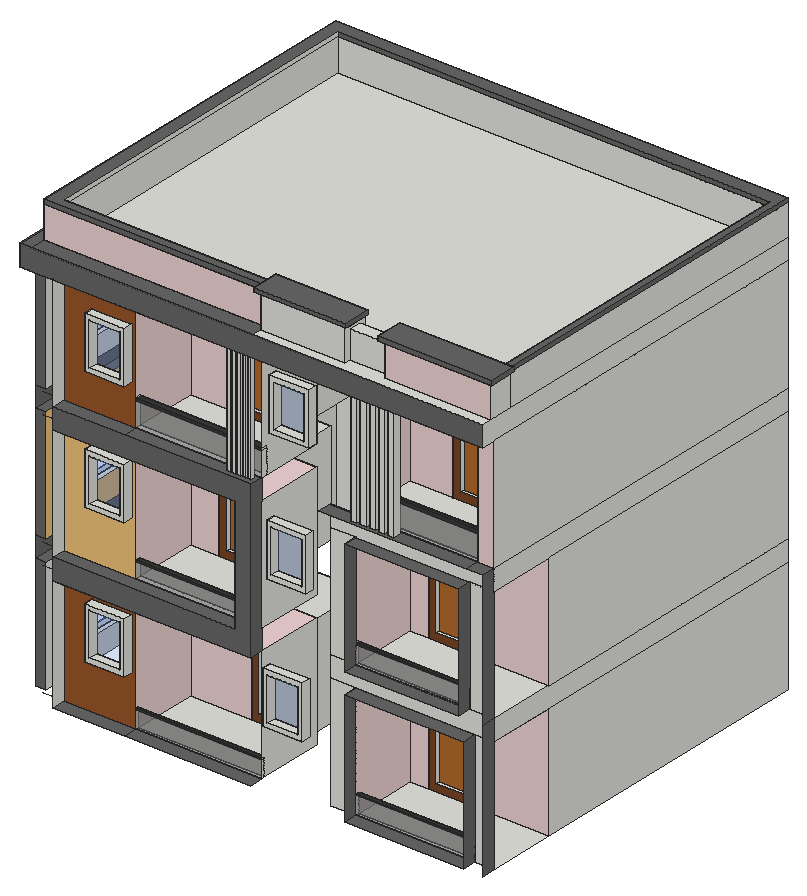
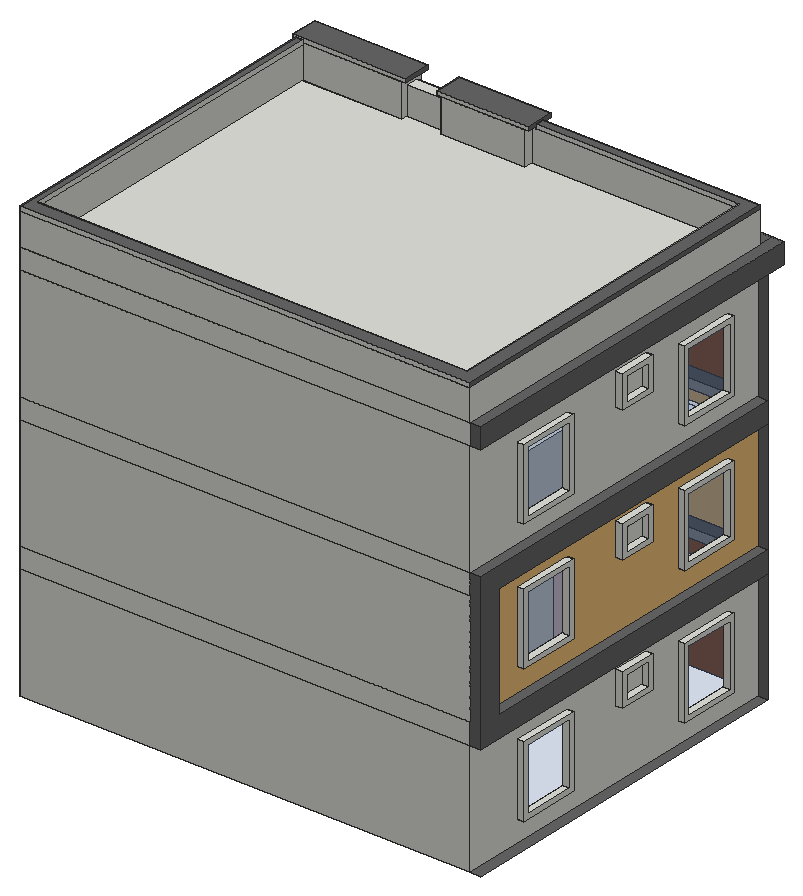
# SketchUp Ruby script. Lengths in inches.
U = 1.inch
M = Sketchup.active_model
def pt(a) = Geom::Point3d.new(a.map { |v| v * U })
def face(e, loops, mat)
  f = e.add_face(loops[0].map { |a| pt(a) })
  loops[1..].each { |l| e.add_face(l.map { |a| pt(a) }).erase! }
  f.material = f.back_material = mat if mat
  f
end
# faces: each face lists its corners as indices into pts; further lists are holes
def faces(e, pts, list, mat = nil) = list.each { |f| face(e, (f[0].is_a?(Array) ? f : [f]).map { |l| l.map { |i| pts[i] } }, mat) }
# xy, xz, yz: faces in a plane at the given z, y or x. An outline is a flat list of corners, or four numbers for a rectangle; further outlines are holes
def ring(l) = l.size == 4 ? [[l[0], l[1]], [l[2], l[1]], [l[2], l[3]], [l[0], l[3]]] : l.each_slice(2).to_a
def flat(e, list, mat, &to3) = list.each { |f| face(e, (f[0].is_a?(Array) ? f : [f]).map { |l| ring(l).map { |u, v| to3.(u, v) } }, mat) }
def xy(e, z, list, mat = nil) = flat(e, list, mat) { |x, y| [x, y, z] }
def xz(e, y, list, mat = nil) = flat(e, list, mat) { |x, z| [x, y, z] }
def yz(e, x, list, mat = nil) = flat(e, list, mat) { |y, z| [x, y, z] }
def lines(e, pts, list) = list.each { |a, b| e.add_line(pt(pts[a]), pt(pts[b])) }
# prism: a flat outline (further loops are holes) pulled along v
def prism(e, loops, v, mat = nil)
  f = face(e, loops, mat); d = Geom::Vector3d.new(v.map { |x| x * U })
  f.pushpull(f.normal.samedirection?(d) ? d.length : -d.length)
end
def box(e, o, s, mat = nil) = prism(e, [[o, [o[0] + s[0], o[1], o[2]], [o[0] + s[0], o[1] + s[1], o[2]], [o[0], o[1] + s[1], o[2]]]], [0, 0, s[2]], mat)
def at(x, y, z, deg = 0) = Geom::Transformation.translation(pt([x, y, z])) * Geom::Transformation.rotation(ORIGIN, Z_AXIS, deg.degrees)
def axes(o, x, y, z) = Geom::Transformation.new([*x, 0, *y, 0, *z, 0, *pt(o).to_a, 1])
def part(name) = M.definitions.add(name)
# library, detail: a bought-in or finely detailed component or shape, given as its bounding box
def library(name, o, s) = part(name).tap { |d| box(d.entities, o, s) }
def detail(e, o, s) = box(e.add_group.entities, o, s)
def put(e, d, t, mat = nil) = e.add_instance(d, t).tap { |i| i.material = mat if mat }
def group(e, t, mat = nil) = e.add_group.tap { |g| g.transformation = t; g.material = mat if mat }.entities
root = M.entities
M.materials.add("Generic").color = [103, 103, 103]
M.materials.add("Generic\#1").color = [239, 210, 210]
M.materials.add("[Color M07]").color = [58, 58, 58]
M.materials.add("[Translucent Glass Blue]").color = [98, 147, 234]
M.materials["[Translucent Glass Blue]"].alpha = 0.25
M.materials.add("[Translucent Glass Gray]").color = [128, 128, 128]
M.materials["[Translucent Glass Gray]"].alpha = 0.5
M.materials.add("[Wood Bamboo]").color = [177, 105, 43]
M.materials.add("[Wood Cherry Original]").color = [152, 86, 42]
M.materials.add("[Wood OSB]").color = [240, 195, 122]
M.materials.add("[Wood Veneer 01]").color = [120, 70, 37]
c1 = part("Group\#1")
xy(c1.entities,0,[[0,0,76.25,8.9375]])
xy(c1.entities,11.01,[[11.01,0,65.24,5.9375]])
xy(c1.entities,138.8,[[11.01,0,65.24,5.9375]])
xy(c1.entities,149.8125,[[0,0,76.25,8.9375]])
xz(c1.entities,0,[[[0,0,76.25,149.8125],[11.01,11.01,65.24,138.8]]],"[Wood Veneer 01]")
xz(c1.entities,5.9375,[[11.01,11.01,65.24,138.8]],"[Wood Bamboo]")
xz(c1.entities,8.9375,[[0,0,76.25,149.8125]])
yz(c1.entities,0,[[0,0,8.9375,149.8125]])
yz(c1.entities,11.01,[[0,11.01,5.9375,138.8]])
yz(c1.entities,65.24,[[0,11.01,5.9375,138.8]])
yz(c1.entities,76.25,[[0,0,8.9375,149.8125]])
xy(root,595.875,[[461.64,66.43,647.41,70.56],[785.17,66.43,960.48,72.06],[960.48,66.43,960.48,72.06,785.17,72.06,785.17,167.12,989.0625,167.12,989.0625,66.43],[461.64,70.56,461.64,167.12,551.875,167.12,551.875,277.93,628.125,277.93,628.125,167.12,647.41,167.12,647.41,70.56],[812,167.12,888.25,277.93]])
xy(root,595.875,[[356.25,45.93,461.64,66.43],[461.64,45.93,647.41,66.43],[785.17,45.93,960.48,66.43],[307.875,73.93,323.875,606.43]],"Generic")
xy(root,621.1875,[[461.64,66.43,647.41,70.56]])
xy(root,622.3125,[[785.17,66.43,960.48,72.06]])
xy(root,623.75,[[461.64,66.43,647.41,70.56]],"[Color M07]")
xy(root,624.6875,[[785.17,66.43,960.48,72.06]],"[Color M07]")
xy(root,627.86,[[313.8125,129.65,323.875,221.17],[313.8125,426.9,323.875,518.42]])
xy(root,634.68,[[313.8125,136.47,323.875,214.35],[313.8125,433.72,323.875,511.6]])
xy(root,668.22,[[397.09,53.18,455.09,66.43]])
xy(root,674.73,[[403.59,53.18,448.59,66.43]])
xy(root,675.14,[[659.17,53.18,717.17,66.43]])
xy(root,681.64,[[665.67,53.18,710.67,66.43]])
xy(root,698.74,[[312.6875,281.29,323.875,336.99]])
xy(root,705.5625,[[312.6875,288.11,323.875,330.17]])
xy(root,726.68,[[313.8125,136.47,323.875,214.35],[313.8125,433.72,323.875,511.6]])
xy(root,733.5,[[313.8125,129.65,323.875,221.17],[313.8125,426.9,323.875,518.42]])
xy(root,738.35,[[403.59,53.18,448.59,66.43]])
xy(root,740.25,[[312.6875,288.11,323.875,330.17]])
xy(root,744.6875,[[551.875,167.12,628.125,277.93],[812,167.12,888.25,277.93]])
xy(root,744.85,[[397.09,53.18,455.09,66.43]])
xy(root,745.27,[[665.67,53.18,710.67,66.43]])
xy(root,747.07,[[312.6875,281.29,323.875,336.99]])
xy(root,751.77,[[659.17,53.18,717.17,66.43]])
xy(root,763.875,[[356.25,45.93,647.41,66.43],[785.17,45.93,960.48,66.43],[307.875,73.93,323.875,606.43]],"Generic")
xy(root,763.875,[[461.64,66.43,647.41,167.12],[785.17,66.43,989.0625,167.12]],"Generic\#1")
xy(root,794.5,[[461.64,66.43,623.41,73.18],[623.41,66.43,623.41,73.18,461.64,73.18,461.64,167.12,503.75,167.12,503.75,277.93,580,277.93,580,167.12,647.41,167.12,647.41,66.43],[785.17,66.43,952.9375,71.18],[952.9375,66.43,952.9375,71.18,785.17,71.18,785.17,167.12,812,167.12,812,277.93,888.25,277.93,888.25,167.12,989.0625,167.12,989.0625,66.43]])
xy(root,794.5,[[356.25,45.93,623.41,66.43],[785.17,45.93,952.9375,66.43],[307.875,73.93,323.875,571.93]],"Generic")
xy(root,816,[[461.64,66.43,623.41,73.18]])
xy(root,819,[[461.64,66.43,623.41,73.18]],"[Color M07]")
xy(root,820.9375,[[785.17,66.43,952.9375,71.18]])
xy(root,823.3125,[[785.17,66.43,952.9375,71.18]],"[Color M07]")
xy(root,830.36,[[313.8125,129.65,323.875,221.17],[313.8125,426.9,323.875,518.42]])
xy(root,837.18,[[313.8125,136.47,323.875,214.35],[313.8125,433.72,323.875,511.6]])
xy(root,871.85,[[397.09,53.18,455.09,66.43],[664.84,53.18,722.84,66.43]])
xy(root,878.35,[[403.59,53.18,448.59,66.43],[671.34,53.18,716.34,66.43]])
xy(root,895.49,[[312.6875,281.29,323.875,336.99]])
xy(root,902.3125,[[312.6875,288.11,323.875,330.17]])
xy(root,929.18,[[313.8125,136.47,323.875,214.35],[313.8125,433.72,323.875,511.6]])
xy(root,936,[[313.8125,129.65,323.875,221.17],[313.8125,426.9,323.875,518.42]])
xy(root,937,[[312.6875,288.11,323.875,330.17]])
xy(root,941.98,[[403.59,53.18,448.59,66.43],[671.34,53.18,716.34,66.43]])
xy(root,943.82,[[312.6875,281.29,323.875,336.99]])
xy(root,944.3125,[[503.75,167.12,580,277.93],[812,167.12,888.25,277.93]])
xy(root,948.48,[[397.09,53.18,455.09,66.43],[664.84,53.18,722.84,66.43]])
xy(root,962.5,[[356.25,45.93,461.64,66.43],[461.64,45.93,623.41,66.43],[785.17,45.93,952.9375,66.43],[307.875,73.93,323.875,571.93]],"Generic")
xy(root,962.5,[[461.64,66.43,647.41,167.12],[785.17,66.43,989.0625,167.12]],"Generic\#1")
xy(root,993.125,[[461.64,66.43,647.41,74.74],[785.17,66.43,965.0625,71.74],[785.17,71.74,965.0625,167.12],[461.64,74.74,461.64,167.12,530.87,167.12,530.87,277.93,607.12,277.93,607.12,167.12,647.41,167.12,647.41,74.74],[848.37,167.12,924.62,277.93]])
xy(root,993.125,[[356.25,45.93,461.64,66.43],[[461.64,45.93,647.41,66.43],[635.77,54.52,641.21,59.96],[628.08,54.52,633.52,59.96],[620.39,54.52,625.83,59.96],[612.71,54.52,618.14,59.96],[605.02,54.52,610.46,59.96]],[[748.05,45.93,965.0625,66.43],[790.64,51.09,800.01,62.22],[804.2,51.09,813.58,62.22],[817.76,51.09,827.14,62.22],[831.33,51.09,840.7,62.22],[844.89,51.09,854.26,62.22]],[965.0625,45.93,989.0625,66.43],[307.875,73.93,323.875,606.43]],"Generic")
xy(root,1022.3,[[313.8125,129.65,323.875,221.17],[313.8125,426.9,323.875,518.42]])
xy(root,1028.5,[[461.64,66.43,647.41,74.74]])
xy(root,1029.12,[[313.8125,136.47,323.875,214.35],[313.8125,433.72,323.875,511.6]])
xy(root,1030.25,[[785.17,66.43,965.0625,71.74]])
xy(root,1032.5625,[[461.64,66.43,647.41,74.74]],"[Color M07]")
xy(root,1035.25,[[785.17,66.43,965.0625,71.74]],"[Color M07]")
xy(root,1050.97,[[397.09,53.18,455.09,66.43]])
xy(root,1057.48,[[403.59,53.18,448.59,66.43]])
xy(root,1064.99,[[668.28,53.18,726.28,66.43]])
xy(root,1071.5,[[674.78,53.18,719.78,66.43]])
xy(root,1094.49,[[312.6875,281.29,323.875,336.99]])
xy(root,1101.3125,[[312.6875,288.11,323.875,330.17]])
xy(root,1121.1,[[403.59,53.18,448.59,66.43]])
xy(root,1121.12,[[313.8125,136.47,323.875,214.35],[313.8125,433.72,323.875,511.6]])
xy(root,1127.6,[[397.09,53.18,455.09,66.43]])
xy(root,1127.9375,[[313.8125,129.65,323.875,221.17],[313.8125,426.9,323.875,518.42]])
xy(root,1135.12,[[674.78,53.18,719.78,66.43]])
xy(root,1136,[[312.6875,288.11,323.875,330.17]])
xy(root,1141.625,[[668.28,53.18,726.28,66.43]])
xy(root,1142.82,[[312.6875,281.29,323.875,336.99]])
xy(root,1142.9375,[[530.87,167.12,607.12,277.93],[848.37,167.12,924.62,277.93]])
xy(root,1161.125,[[307.875,45.93,323.875,73.93],[323.875,45.93,323.875,606.43,989.0625,606.43,989.0625,66.43,965.0625,66.43,965.0625,167.12,785.17,167.12,785.17,66.43,647.41,66.43,647.41,167.12,461.64,167.12,461.64,66.43,356.25,66.43,356.25,45.93],[790.64,45.93,800.01,51.09],[804.2,45.93,813.58,51.09],[817.76,45.93,827.14,51.09],
  [831.33,45.93,840.7,51.09],[844.89,45.93,854.26,51.09],[965.0625,45.93,989.0625,66.43],[790.64,51.09,800.01,62.22],[804.2,51.09,813.58,62.22],
  [817.76,51.09,827.14,62.22],[831.33,51.09,840.7,62.22],[844.89,51.09,854.26,62.22]])
xy(root,1161.125,[[356.25,45.93,461.64,66.43],[647.41,45.93,785.17,66.43],[307.875,73.93,323.875,606.43]],"Generic")
xy(root,1161.125,[[[461.64,45.93,647.41,167.12],[635.77,54.52,641.21,59.96],[628.08,54.52,633.52,59.96],[620.39,54.52,625.83,59.96],[612.71,54.52,618.14,59.96],[605.02,54.52,610.46,59.96]],[785.17,45.93,785.17,167.12,965.0625,167.12,965.0625,45.93,854.26,45.93,854.26,62.22,844.89,62.22,844.89,45.93,840.7,45.93,840.7,62.22,831.33,62.22,831.33,45.93,827.14,45.93,827.14,62.22,817.76,62.22,817.76,45.93,813.58,45.93,813.58,62.22,804.2,62.22,804.2,45.93,800.01,45.93,800.01,62.22,790.64,62.22,790.64,45.93]],"Generic\#1")
xy(root,1191.75,[[650.17,45.93,650.17,60.43,774.86,60.43,774.86,68.81,832.36,68.81,832.36,60.43,989.0625,60.43,989.0625,45.93],[650.17,60.43,774.86,95.68],[832.36,60.43,989.0625,95.68],[774.86,68.81,832.36,69.93],[323.875,69.93,323.875,606.43,989.0625,606.43,989.0625,95.68,979.4375,95.68,979.4375,586.43,343.5625,586.43,343.5625,82.81,650.17,82.81,650.17,69.93],
  [774.86,69.93,832.36,87.3],[343.5625,82.81,650.17,82.81,650.17,95.68,774.86,95.68,774.86,87.3,832.36,87.3,832.36,95.68,979.4375,95.68,979.4375,586.43,343.5625,586.43]])
xy(root,1191.75,[[307.875,45.93,323.875,606.43],[323.875,45.93,650.17,69.93]],"Generic")
xy(root,1233.18,[[774.86,68.81,832.36,87.3]])
xy(root,1238.5625,[[323.875,69.93,323.875,606.43,989.0625,606.43,989.0625,95.68,979.4375,95.68,979.4375,586.43,343.5625,586.43,343.5625,82.81,644.54,82.81,644.54,69.93]])
xy(root,1241.5625,[[644.54,54.81,780.49,60.43],[826.74,54.81,994.6875,60.43],[644.54,60.43,650.17,69.93],[650.17,60.43,774.86,95.68],[774.86,60.43,780.49,95.68],
  [826.74,60.43,832.36,95.68],[832.36,60.43,989.0625,95.68],[989.0625,60.43,994.6875,95.68],[644.54,69.93,650.17,82.81],[644.54,82.81,650.17,95.68]])
xy(root,1245.25,[[323.875,69.93,644.54,69.93,644.54,82.81,343.5625,82.81,343.5625,586.43,979.4375,586.43,979.4375,95.68,989.0625,95.68,989.0625,606.43,323.875,606.43]],"Generic")
xy(root,1247.6875,[[644.54,54.81,780.49,95.68],[826.74,54.81,994.6875,95.68]],"Generic")
xz(root,45.93,[[356.25,763.875,647.41,763.875,647.41,993.125,356.25,993.125,356.25,962.5,623.41,962.5,623.41,794.5,356.25,794.5],[307.875,1161.125,989.0625,1191.75]],"Generic")
xz(root,51.09,[[790.64,993.125,800.01,1161.125],[804.2,993.125,813.58,1161.125],[817.76,993.125,827.14,1161.125],[831.33,993.125,840.7,1161.125],[844.89,993.125,854.26,1161.125]])
xz(root,53.18,[[[397.09,668.22,455.09,744.85],[403.59,674.73,448.59,738.35]],[[659.17,675.14,717.17,751.77],[665.67,681.64,710.67,745.27]],[[397.09,871.85,455.09,948.48],[403.59,878.35,448.59,941.98]],[[664.84,871.85,722.84,948.48],[671.34,878.35,716.34,941.98]],[[397.09,1050.97,455.09,1127.6],[403.59,1057.48,448.59,1121.1]],
  [[668.28,1064.99,726.28,1141.625],[674.78,1071.5,719.78,1135.12]]])
xz(root,54.52,[[605.02,993.125,610.46,1161.125],[612.71,993.125,618.14,1161.125],[620.39,993.125,625.83,1161.125],[628.08,993.125,633.52,1161.125],[635.77,993.125,641.21,1161.125]])
xz(root,54.81,[[644.54,1241.5625,780.49,1247.6875],[826.74,1241.5625,994.6875,1247.6875]],"Generic")
xz(root,59.96,[[605.02,993.125,610.46,1161.125],[612.71,993.125,618.14,1161.125],[620.39,993.125,625.83,1161.125],[628.08,993.125,633.52,1161.125],[635.77,993.125,641.21,1161.125]])
xz(root,60.43,[[650.17,1191.75,774.86,1241.5625]])
xz(root,60.43,[[832.36,1191.75,989.0625,1241.5625]],"Generic\#1")
xz(root,62.22,[[790.64,993.125,800.01,1161.125],[804.2,993.125,813.58,1161.125],[817.76,993.125,827.14,1161.125],[831.33,993.125,840.7,1161.125],[844.89,993.125,854.26,1161.125]])
xz(root,66.43,[[748.05,595.875,785.17,763.875],[960.48,595.875,989.0625,763.875],[748.05,763.875,989.0625,794.5],[623.41,794.5,647.41,962.5],[748.05,794.5,785.17,962.5],
  [952.9375,794.5,989.0625,962.5],[748.05,962.5,989.0625,993.125]])
xz(root,66.43,[[965.0625,993.125,989.0625,1161.125]],"Generic\#1")
xz(root,66.43,[[461.64,621.1875,647.41,623.75],[785.17,622.3125,960.48,624.6875],[461.64,816,623.41,819],[785.17,820.9375,952.9375,823.3125],[461.64,1028.5,647.41,1032.5625],
  [785.17,1030.25,965.0625,1035.25]],"[Color M07]")
xz(root,66.43,[[403.59,674.73,448.59,738.35],[665.67,681.64,710.67,745.27],[403.59,878.35,448.59,941.98],[671.34,878.35,716.34,941.98],[403.59,1057.48,448.59,1121.1],
  [674.78,1071.5,719.78,1135.12]],"[Translucent Glass Blue]")
xz(root,66.43,[[461.64,595.875,647.41,621.1875],[785.17,595.875,960.48,622.3125],[461.64,794.5,623.41,816],[785.17,794.5,952.9375,820.9375],[461.64,993.125,647.41,1028.5],
  [785.17,993.125,965.0625,1030.25]],"[Translucent Glass Gray]")
xz(root,66.43,[[[356.25,595.875,461.64,763.875],[397.09,668.22,455.09,744.85]],[[356.25,993.125,461.64,1161.125],[397.09,1050.97,455.09,1127.6]]],"[Wood Cherry Original]")
xz(root,66.43,[[[356.25,794.5,461.64,962.5],[397.09,871.85,455.09,948.48]]],"[Wood OSB]")
xz(root,68.81,[[774.86,1191.75,832.36,1233.18]])
xz(root,69.93,[[323.875,1238.5625,644.54,1245.25]],"Generic")
xz(root,69.93,[[323.875,1191.75,650.17,1191.75,650.17,1241.5625,644.54,1241.5625,644.54,1238.5625,323.875,1238.5625]],"Generic\#1")
xz(root,70.56,[[461.64,621.1875,647.41,623.75]])
xz(root,70.56,[[461.64,595.875,647.41,621.1875]],"[Translucent Glass Gray]")
xz(root,71.18,[[785.17,820.9375,952.9375,823.3125]])
xz(root,71.18,[[785.17,794.5,952.9375,820.9375]],"[Translucent Glass Gray]")
xz(root,71.74,[[785.17,1030.25,965.0625,1035.25]])
xz(root,71.74,[[785.17,993.125,965.0625,1030.25]],"[Translucent Glass Gray]")
xz(root,72.06,[[785.17,622.3125,960.48,624.6875]])
xz(root,72.06,[[785.17,595.875,960.48,622.3125]],"[Translucent Glass Gray]")
xz(root,73.18,[[461.64,816,623.41,819]])
xz(root,73.18,[[461.64,794.5,623.41,816]],"[Translucent Glass Gray]")
xz(root,73.93,[[307.875,595.875,323.875,763.875],[307.875,794.5,323.875,962.5],[307.875,993.125,323.875,1161.125]],"Generic")
xz(root,74.74,[[461.64,1028.5,647.41,1032.5625]])
xz(root,74.74,[[461.64,993.125,647.41,1028.5]],"[Translucent Glass Gray]")
xz(root,82.81,[[343.5625,1191.75,343.5625,1238.5625,644.54,1238.5625,644.54,1241.5625,650.17,1241.5625,650.17,1191.75],[343.5625,1238.5625,644.54,1245.25]])
xz(root,87.3,[[774.86,1191.75,832.36,1233.18]])
xz(root,95.68,[[650.17,1191.75,774.86,1241.5625],[832.36,1191.75,979.4375,1241.5625],[979.4375,1238.5625,989.0625,1241.5625],[644.54,1241.5625,780.49,1247.6875],[826.74,1241.5625,826.74,1247.6875,994.6875,1247.6875,994.6875,1241.5625,989.0625,1241.5625,989.0625,1245.25,979.4375,1245.25,979.4375,1241.5625],
  [979.4375,1241.5625,989.0625,1245.25]])
xz(root,129.65,[[313.8125,627.86,323.875,733.5],[313.8125,830.36,323.875,936],[313.8125,1022.3,323.875,1127.9375]])
xz(root,136.47,[[313.8125,634.68,323.875,726.68],[313.8125,837.18,323.875,929.18],[313.8125,1029.12,323.875,1121.12]])
xz(root,167.12,[[848.37,974.55,924.62,993.125]])
xz(root,167.12,[[461.64,595.875,551.875,595.875,551.875,744.6875,628.125,744.6875,628.125,595.875,647.41,595.875,647.41,763.875,461.64,763.875],[785.17,595.875,812,595.875,812,744.6875,888.25,744.6875,888.25,595.875,989.0625,595.875,989.0625,763.875,785.17,763.875],[461.64,794.5,503.75,794.5,503.75,944.3125,580,944.3125,580,794.5,647.41,794.5,647.41,962.5,461.64,962.5],[785.17,794.5,812,794.5,812,944.3125,888.25,944.3125,888.25,794.5,989.0625,794.5,989.0625,962.5,785.17,962.5],[461.64,993.125,530.87,993.125,530.87,1142.9375,607.12,1142.9375,607.12,993.125,647.41,993.125,647.41,1161.125,461.64,1161.125],
  [785.17,993.125,848.37,993.125,848.37,1142.9375,924.62,1142.9375,924.62,993.125,965.0625,993.125,965.0625,1161.125,785.17,1161.125]],"Generic\#1")
xz(root,214.35,[[313.8125,634.68,323.875,726.68],[313.8125,837.18,323.875,929.18],[313.8125,1029.12,323.875,1121.12]])
xz(root,221.17,[[313.8125,627.86,323.875,733.5],[313.8125,830.36,323.875,936],[313.8125,1022.3,323.875,1127.9375]])
xz(root,277.93,[[551.875,595.875,628.125,744.6875],[812,595.875,888.25,744.6875],[503.75,794.5,580,944.3125],[812,794.5,888.25,944.3125],[530.87,993.125,607.12,1142.9375],
  [848.37,993.125,924.62,1142.9375]])
xz(root,281.29,[[312.6875,698.74,323.875,747.07],[312.6875,895.49,323.875,943.82],[312.6875,1094.49,323.875,1142.82]])
xz(root,288.11,[[312.6875,705.5625,323.875,740.25],[312.6875,902.3125,323.875,937],[312.6875,1101.3125,323.875,1136]])
xz(root,330.17,[[312.6875,705.5625,323.875,740.25],[312.6875,902.3125,323.875,937],[312.6875,1101.3125,323.875,1136]])
xz(root,336.99,[[312.6875,698.74,323.875,747.07],[312.6875,895.49,323.875,943.82],[312.6875,1094.49,323.875,1142.82]])
xz(root,426.9,[[313.8125,627.86,323.875,733.5],[313.8125,830.36,323.875,936],[313.8125,1022.3,323.875,1127.9375]])
xz(root,433.72,[[313.8125,634.68,323.875,726.68],[313.8125,837.18,323.875,929.18],[313.8125,1029.12,323.875,1121.12]])
xz(root,511.6,[[313.8125,634.68,323.875,726.68],[313.8125,837.18,323.875,929.18],[313.8125,1029.12,323.875,1121.12]])
xz(root,518.42,[[313.8125,627.86,323.875,733.5],[313.8125,830.36,323.875,936],[313.8125,1022.3,323.875,1127.9375]])
xz(root,571.93,[[307.875,794.5,323.875,962.5]],"Generic")
xz(root,586.43,[[343.5625,1191.75,979.4375,1238.5625]])
xz(root,586.43,[[343.5625,1238.5625,979.4375,1245.25]],"Generic")
xz(root,606.43,[[323.875,595.875,989.0625,763.875],[323.875,763.875,989.0625,794.5],[323.875,794.5,989.0625,962.5],[323.875,962.5,989.0625,993.125],[323.875,993.125,989.0625,1161.125],
  [323.875,1161.125,989.0625,1191.75],[323.875,1191.75,989.0625,1238.5625],[323.875,1238.5625,989.0625,1245.25]])
xz(root,606.43,[[307.875,763.875,323.875,993.125],[307.875,1161.125,323.875,1191.75]],"Generic")
yz(root,307.875,[[73.93,763.875,73.93,794.5,571.93,794.5,571.93,962.5,73.93,962.5,73.93,993.125,606.43,993.125,606.43,763.875],[45.93,1161.125,606.43,1191.75]],"Generic")
yz(root,312.6875,[[[281.29,698.74,336.99,747.07],[288.11,705.5625,330.17,740.25]],[[281.29,895.49,336.99,943.82],[288.11,902.3125,330.17,937]],[[281.29,1094.49,336.99,1142.82],[288.11,1101.3125,330.17,1136]]])
yz(root,313.8125,[[[129.65,627.86,221.17,733.5],[136.47,634.68,214.35,726.68]],[[426.9,627.86,518.42,733.5],[433.72,634.68,511.6,726.68]],[[129.65,830.36,221.17,936],[136.47,837.18,214.35,929.18]],[[426.9,830.36,518.42,936],[433.72,837.18,511.6,929.18]],[[129.65,1022.3,221.17,1127.9375],[136.47,1029.12,214.35,1121.12]],
  [[426.9,1022.3,518.42,1127.9375],[433.72,1029.12,511.6,1121.12]]])
yz(root,323.875,[[[73.93,595.875,606.43,763.875],[129.65,627.86,221.17,733.5],[426.9,627.86,518.42,733.5],[281.29,698.74,336.99,747.07]],[288.11,705.5625,330.17,740.25],[288.11,902.3125,330.17,937],[[73.93,993.125,606.43,1161.125],[129.65,1022.3,221.17,1127.9375],[426.9,1022.3,518.42,1127.9375],[281.29,1094.49,336.99,1142.82]],[288.11,1101.3125,330.17,1136],
  [69.93,1191.75,606.43,1238.5625]])
yz(root,323.875,[[69.93,1238.5625,606.43,1245.25]],"Generic")
yz(root,323.875,[[136.47,634.68,214.35,726.68],[433.72,634.68,511.6,726.68],[136.47,837.18,214.35,929.18],[433.72,837.18,511.6,929.18],[136.47,1029.12,214.35,1121.12],
  [433.72,1029.12,511.6,1121.12]],"[Translucent Glass Blue]")
yz(root,323.875,[[[73.93,794.5,571.93,962.5],[129.65,830.36,221.17,936],[426.9,830.36,518.42,936],[281.29,895.49,336.99,943.82]]],"[Wood OSB]")
yz(root,343.5625,[[82.81,1191.75,586.43,1238.5625],[82.81,1238.5625,586.43,1245.25]])
yz(root,356.25,[[45.93,595.875,66.43,763.875],[45.93,794.5,66.43,962.5],[45.93,993.125,66.43,1161.125]])
yz(root,397.09,[[53.18,668.22,66.43,744.85],[53.18,871.85,66.43,948.48],[53.18,1050.97,66.43,1127.6]])
yz(root,403.59,[[53.18,674.73,66.43,738.35],[53.18,878.35,66.43,941.98],[53.18,1057.48,66.43,1121.1]])
yz(root,448.59,[[53.18,674.73,66.43,738.35],[53.18,878.35,66.43,941.98],[53.18,1057.48,66.43,1121.1]])
yz(root,455.09,[[53.18,668.22,66.43,744.85],[53.18,871.85,66.43,948.48],[53.18,1050.97,66.43,1127.6]])
yz(root,461.64,[[66.43,595.875,70.56,621.1875],[66.43,621.1875,70.56,623.75],[66.43,794.5,73.18,816],[66.43,816,73.18,819],[66.43,993.125,74.74,1028.5],
  [66.43,1028.5,74.74,1032.5625]])
yz(root,461.64,[[70.56,595.875,167.12,595.875,167.12,763.875,66.43,763.875,66.43,623.75,70.56,623.75],[73.18,794.5,167.12,794.5,167.12,962.5,66.43,962.5,66.43,819,73.18,819],[74.74,993.125,167.12,993.125,167.12,1161.125,66.43,1161.125,66.43,1032.5625,74.74,1032.5625]],"Generic\#1")
yz(root,503.75,[[167.12,794.5,277.93,944.3125]])
yz(root,530.87,[[167.12,993.125,277.93,1142.9375]])
yz(root,551.875,[[167.12,595.875,277.93,744.6875]])
yz(root,580,[[167.12,794.5,277.93,944.3125]])
yz(root,605.02,[[54.52,993.125,59.96,1161.125]])
yz(root,607.12,[[167.12,993.125,277.93,1142.9375]])
yz(root,610.46,[[54.52,993.125,59.96,1161.125]])
yz(root,612.71,[[54.52,993.125,59.96,1161.125]])
yz(root,618.14,[[54.52,993.125,59.96,1161.125]])
yz(root,620.39,[[54.52,993.125,59.96,1161.125]])
yz(root,623.41,[[66.43,794.5,73.18,816],[66.43,816,73.18,819]])
yz(root,623.41,[[45.93,794.5,66.43,962.5]],"Generic")
yz(root,625.83,[[54.52,993.125,59.96,1161.125]])
yz(root,628.08,[[54.52,993.125,59.96,1161.125]])
yz(root,628.125,[[167.12,595.875,277.93,744.6875]])
yz(root,633.52,[[54.52,993.125,59.96,1161.125]])
yz(root,635.77,[[54.52,993.125,59.96,1161.125]])
yz(root,641.21,[[54.52,993.125,59.96,1161.125]])
yz(root,644.54,[[69.93,1238.5625,82.81,1241.5625]])
yz(root,644.54,[[54.81,1241.5625,54.81,1247.6875,95.68,1247.6875,95.68,1241.5625,82.81,1241.5625,82.81,1245.25,69.93,1245.25,69.93,1241.5625],[69.93,1241.5625,82.81,1245.25]],"Generic")
yz(root,647.41,[[66.43,595.875,70.56,621.1875],[70.56,595.875,70.56,623.75,66.43,623.75,66.43,763.875,167.12,763.875,167.12,595.875],[66.43,621.1875,70.56,623.75],[66.43,794.5,167.12,962.5],[66.43,993.125,74.74,1028.5],
  [74.74,993.125,74.74,1032.5625,66.43,1032.5625,66.43,1161.125,167.12,1161.125,167.12,993.125],[66.43,1028.5,74.74,1032.5625]])
yz(root,647.41,[[45.93,763.875,66.43,993.125]],"Generic")
yz(root,650.17,[[60.43,1191.75,69.93,1241.5625],[69.93,1191.75,82.81,1241.5625],[82.81,1191.75,95.68,1241.5625]])
yz(root,659.17,[[53.18,675.14,66.43,751.77]])
yz(root,664.84,[[53.18,871.85,66.43,948.48]])
yz(root,665.67,[[53.18,681.64,66.43,745.27]])
yz(root,668.28,[[53.18,1064.99,66.43,1141.625]])
yz(root,671.34,[[53.18,878.35,66.43,941.98]])
yz(root,674.78,[[53.18,1071.5,66.43,1135.12]])
yz(root,710.67,[[53.18,681.64,66.43,745.27]])
yz(root,716.34,[[53.18,878.35,66.43,941.98]])
yz(root,717.17,[[53.18,675.14,66.43,751.77]])
yz(root,719.78,[[53.18,1071.5,66.43,1135.12]])
yz(root,722.84,[[53.18,871.85,66.43,948.48]])
yz(root,726.28,[[53.18,1064.99,66.43,1141.625]])
yz(root,774.86,[[60.43,1191.75,68.81,1191.75,68.81,1233.18,87.3,1233.18,87.3,1191.75,95.68,1191.75,95.68,1241.5625,60.43,1241.5625]])
yz(root,780.49,[[54.81,1241.5625,95.68,1247.6875]],"Generic")
yz(root,785.17,[[66.43,595.875,72.06,622.3125],[66.43,622.3125,72.06,624.6875],[66.43,794.5,71.18,820.9375],[66.43,820.9375,71.18,823.3125],[66.43,993.125,71.74,1030.25],
  [66.43,1030.25,71.74,1035.25]])
yz(root,785.17,[[45.93,595.875,66.43,763.875],[45.93,794.5,66.43,962.5]],"Generic")
yz(root,785.17,[[72.06,595.875,167.12,595.875,167.12,763.875,66.43,763.875,66.43,624.6875,72.06,624.6875],[71.18,794.5,167.12,794.5,167.12,962.5,66.43,962.5,66.43,823.3125,71.18,823.3125],[71.74,993.125,167.12,993.125,167.12,1161.125,66.43,1161.125,66.43,1035.25,71.74,1035.25]],"Generic\#1")
yz(root,790.64,[[51.09,993.125,62.22,1161.125]])
yz(root,800.01,[[51.09,993.125,62.22,1161.125]])
yz(root,804.2,[[51.09,993.125,62.22,1161.125]])
yz(root,812,[[167.12,595.875,277.93,744.6875],[167.12,794.5,277.93,944.3125]])
yz(root,813.58,[[51.09,993.125,62.22,1161.125]])
yz(root,817.76,[[51.09,993.125,62.22,1161.125]])
yz(root,826.74,[[54.81,1241.5625,95.68,1247.6875]],"Generic")
yz(root,827.14,[[51.09,993.125,62.22,1161.125]])
yz(root,831.33,[[51.09,993.125,62.22,1161.125]])
yz(root,832.36,[[60.43,1191.75,60.43,1241.5625,95.68,1241.5625,95.68,1191.75,87.3,1191.75,87.3,1233.18,68.81,1233.18,68.81,1191.75]])
yz(root,840.7,[[51.09,993.125,62.22,1161.125]])
yz(root,844.89,[[51.09,993.125,62.22,1161.125]])
yz(root,848.37,[[167.12,993.125,277.93,1142.9375]])
yz(root,854.26,[[51.09,993.125,62.22,1161.125]])
yz(root,888.25,[[167.12,595.875,277.93,744.6875],[167.12,794.5,277.93,944.3125]])
yz(root,924.62,[[167.12,993.125,277.93,1142.9375]])
yz(root,952.9375,[[66.43,794.5,71.18,820.9375],[66.43,820.9375,71.18,823.3125]])
yz(root,952.9375,[[45.93,794.5,66.43,962.5]],"Generic")
yz(root,960.48,[[66.43,595.875,72.06,622.3125],[66.43,622.3125,72.06,624.6875]])
yz(root,960.48,[[45.93,595.875,66.43,763.875]],"Generic")
yz(root,965.0625,[[66.43,993.125,71.74,1030.25],[66.43,1030.25,71.74,1035.25]])
yz(root,965.0625,[[71.74,993.125,71.74,1035.25,66.43,1035.25,66.43,1161.125,167.12,1161.125,167.12,993.125]],"Generic\#1")
yz(root,979.4375,[[95.68,1191.75,586.43,1238.5625],[95.68,1238.5625,586.43,1245.25]])
yz(root,989.0625,[[167.12,595.875,606.43,763.875],[66.43,763.875,606.43,794.5],[167.12,794.5,606.43,962.5],[66.43,962.5,606.43,993.125],[66.43,993.125,606.43,1161.125],
  [45.93,1161.125,606.43,1191.75],[60.43,1191.75,95.68,1241.5625],[95.68,1191.75,606.43,1238.5625]])
yz(root,989.0625,[[45.93,595.875,66.43,794.5],[45.93,794.5,66.43,993.125],[95.68,1238.5625,606.43,1245.25]],"Generic")
yz(root,994.6875,[[54.81,1241.5625,95.68,1247.6875]],"Generic")
p = [[323.875,66.43,595.875],[356.25,66.43,595.875],[323.875,66.43,962.5],[356.25,66.43,962.5],[323.875,66.43,993.125],[356.25,66.43,993.125],
  [960.48,66.43,763.875],[960.48,69.93,763.875],[518.06,167.12,974.55],[594.31,167.12,974.55],[594.31,167.12,993.125],[518.06,167.12,993.125],
  [356.25,66.43,763.875],[323.875,66.43,763.875],[356.25,66.43,794.5],[323.875,66.43,794.5]]
lines(root,p,[[0,1],[2,3],[4,5],[6,7],[8,9],[9,10],[11,8],[12,13],[14,15]])
put(root,c1,at(812,167.12,595.875))
put(root,c1,at(551.875,167.12,595.875))
put(root,c1,at(503.75,167.12,794.5))
put(root,c1,at(812,167.12,794.5))
put(root,c1,at(848.37,167.12,993.125))
put(root,c1,at(530.87,167.12,993.125))
